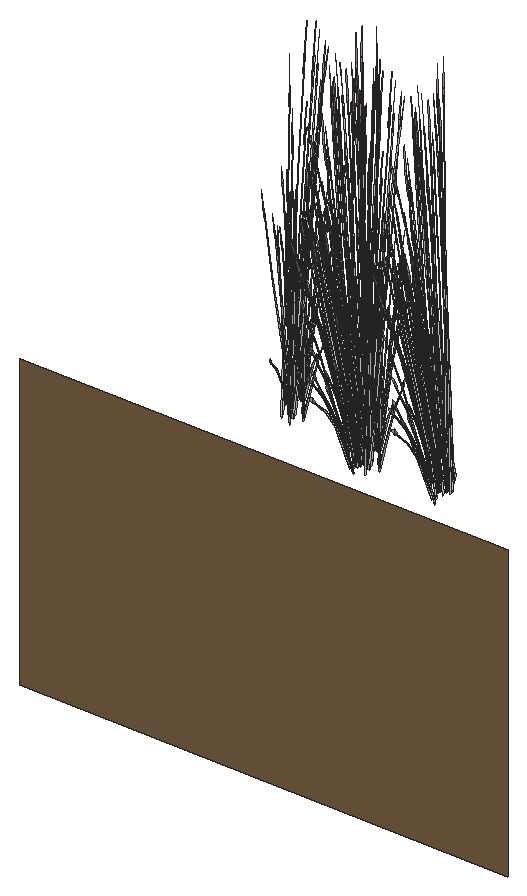
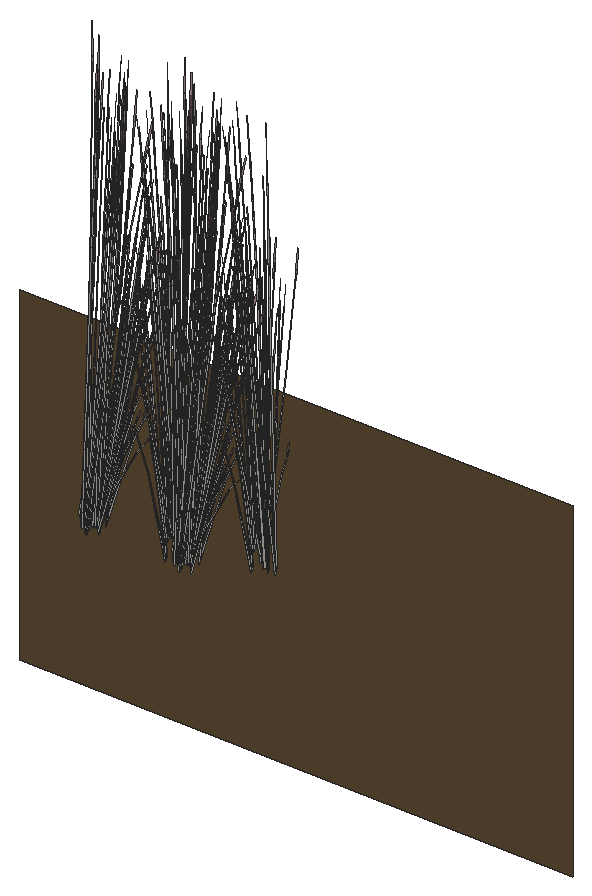
# SketchUp Ruby script. Lengths in inches.
U = 1.inch
M = Sketchup.active_model
def pt(a) = Geom::Point3d.new(a.map { |v| v * U })
def face(e, loops, mat)
  f = e.add_face(loops[0].map { |a| pt(a) })
  loops[1..].each { |l| e.add_face(l.map { |a| pt(a) }).erase! }
  f.material = f.back_material = mat if mat
  f
end
# faces: each face lists its corners as indices into pts; further lists are holes
def faces(e, pts, list, mat = nil) = list.each { |f| face(e, (f[0].is_a?(Array) ? f : [f]).map { |l| l.map { |i| pts[i] } }, mat) }
# xy, xz, yz: faces in a plane at the given z, y or x. An outline is a flat list of corners, or four numbers for a rectangle; further outlines are holes
def ring(l) = l.size == 4 ? [[l[0], l[1]], [l[2], l[1]], [l[2], l[3]], [l[0], l[3]]] : l.each_slice(2).to_a
def flat(e, list, mat, &to3) = list.each { |f| face(e, (f[0].is_a?(Array) ? f : [f]).map { |l| ring(l).map { |u, v| to3.(u, v) } }, mat) }
def xy(e, z, list, mat = nil) = flat(e, list, mat) { |x, y| [x, y, z] }
def xz(e, y, list, mat = nil) = flat(e, list, mat) { |x, z| [x, y, z] }
def yz(e, x, list, mat = nil) = flat(e, list, mat) { |y, z| [x, y, z] }
def lines(e, pts, list) = list.each { |a, b| e.add_line(pt(pts[a]), pt(pts[b])) }
# prism: a flat outline (further loops are holes) pulled along v
def prism(e, loops, v, mat = nil)
  f = face(e, loops, mat); d = Geom::Vector3d.new(v.map { |x| x * U })
  f.pushpull(f.normal.samedirection?(d) ? d.length : -d.length)
end
def box(e, o, s, mat = nil) = prism(e, [[o, [o[0] + s[0], o[1], o[2]], [o[0] + s[0], o[1] + s[1], o[2]], [o[0], o[1] + s[1], o[2]]]], [0, 0, s[2]], mat)
def at(x, y, z, deg = 0) = Geom::Transformation.translation(pt([x, y, z])) * Geom::Transformation.rotation(ORIGIN, Z_AXIS, deg.degrees)
def axes(o, x, y, z) = Geom::Transformation.new([*x, 0, *y, 0, *z, 0, *pt(o).to_a, 1])
def part(name) = M.definitions.add(name)
# library, detail: a bought-in or finely detailed component or shape, given as its bounding box
def library(name, o, s) = part(name).tap { |d| box(d.entities, o, s) }
def detail(e, o, s) = box(e.add_group.entities, o, s)
def put(e, d, t, mat = nil) = e.add_instance(d, t).tap { |i| i.material = mat if mat }
def group(e, t, mat = nil) = e.add_group.tap { |g| g.transformation = t; g.material = mat if mat }.entities
root = M.entities
M.materials.add("LightPink_Translucent").color = [144, 107, 117]
M.materials["LightPink_Translucent"].alpha = 0.75
M.materials.add("Soil_03_1K").color = [122, 96, 67]
c1 = part("blade")
p = [[2.15,0.21,22],[0,0.17,0],[0.09,0.45,0],[2.18,0.31,22],[2.29,0.31,22],[0.38,0.45,0],
  [2.48,0.24,33],[2.49,0.24,33],[2.48,0.22,33]]
faces(c1.entities,p,[[0,1,2,3],[4,5,2,3],[6,3,4,7],[8,0,3,6]])
c2 = part("seeds")
p = [[0.3,-0.1,1.38],[-0.01,-0.03,1.59],[-0.01,-0.03,0.03],[0.14,-0.07,-0.07],[0.29,-0.03,3],[0.15,0.01,3.11]]
faces(c2.entities,p,[[0,1,2,3],[1,0,4,5]],"LightPink_Translucent")
c3 = part("blade with seeds")
put(c3.entities,c1,at(0,0,0))
put(c3.entities,c2,axes([2.4,0.25,30.99],[1.5799,-0.05474,1.17369],[-0.12525,1.92788,0.29478],[-0.07173,-0.02425,1.56792]))
xz(root,0,[[330.57,-48,410.57,0]],"Soil_03_1K")
put(root,c3,axes([368.82,20.52,-9.47],[0.08068,0.14973,1.71376],[-0.3728,0.12606,0.13857],[-0.08426,-0.23506,0.73262]))
put(root,c3,axes([382.24,20.52,-9.33],[0.08068,0.14973,1.71376],[-0.3728,0.12606,0.13857],[-0.08426,-0.23506,0.73262]))
put(root,c3,axes([369.43,19.52,-8.625],[-0.05398,-0.06539,1.74944],[-0.36026,0.04145,-0.27667],[-0.0575,-0.15639,0.14031]))
put(root,c3,axes([382.86,19.52,-8.5],[-0.05398,-0.06539,1.74944],[-0.36026,0.04145,-0.27667],[-0.0575,-0.15639,0.14031]))
put(root,c3,axes([370.27,20.3,-10.75],[-0.10032,0.0944,1.43002],[-0.30046,-0.16522,-0.30754],[0.05569,-0.20547,0.61141]))
put(root,c3,axes([369.8125,20.63,-8.36],[-0.16845,-0.3792,-0.71045],[0.34676,-0.21133,0.08574],[-0.03939,-0.18322,1.00501]))
put(root,c3,axes([383.24,20.63,-8.23],[-0.16845,-0.3792,-0.71045],[0.34676,-0.21133,0.08574],[-0.03939,-0.18322,1.00501]))
put(root,c3,axes([368.72,20.12,-10.75],[-0.02137,0.15256,1.43002],[-0.31245,0.12771,-0.30754],[-0.07303,-0.19719,0.61141]))
put(root,c3,axes([382.14,20.12,-10.62],[-0.02137,0.15256,1.43002],[-0.31245,0.12771,-0.30754],[-0.07303,-0.19719,0.61141]))
put(root,c3,axes([369.52,19.79,-11.85],[-0.0592,0.0168,1.76342],[-0.32738,-0.18913,-0.26939],[0.00549,-0.15776,0.30037]))
put(root,c3,axes([382.95,19.79,-11.72],[-0.0592,0.0168,1.76342],[-0.32738,-0.18913,-0.26939],[0.00549,-0.15776,0.30037]))
put(root,c3,axes([358.04,21,-5.34],[0.00918,-0.43138,-0.71045],[0.38672,0.02897,0.08574],[0.04081,-0.18275,1.00501]))
put(root,c3,axes([370.51,21,-8.36],[0.00918,-0.43138,-0.71045],[0.38672,0.02897,0.08574],[0.04081,-0.18275,1.00501]))
put(root,c3,axes([358.58,20.33,-5.61],[-0.00341,-0.09282,1.74944],[-0.28775,-0.26825,-0.27667],[0.04449,-0.16261,0.14031]))
put(root,c3,axes([371.05,20.33,-8.625],[-0.00341,-0.09282,1.74944],[-0.28775,-0.26825,-0.27667],[0.04449,-0.16261,0.14031]))
put(root,c3,axes([369.84,20.31,-8.82],[0.1064,-0.35863,-0.35414],[0.31043,0.1046,0.4572],[-0.02846,-0.14439,0.87481]))
put(root,c3,axes([383.27,20.31,-8.68],[0.1064,-0.35863,-0.35414],[0.31043,0.1046,0.4572],[-0.02846,-0.14439,0.87481]))
put(root,c3,axes([357.6,20.78,-6.45],[-0.06572,0.16029,1.71376],[-0.27569,-0.33172,0.13857],[0.12437,-0.20675,0.73262]))
put(root,c3,axes([370.08,20.78,-9.47],[-0.06572,0.16029,1.71376],[-0.27569,-0.33172,0.13857],[0.12437,-0.20675,0.73262]))
put(root,c3,axes([370.98,19.99,-8.63],[-0.03584,0.03562,1.77383],[-0.35118,-0.12018,-0.16761],[-0.01271,-0.15545,0.31391]))
put(root,c3,axes([369.6875,20.55,-8.66],[-0.34695,-0.11691,-0.51099],[0.11892,-0.40083,-0.3958],[-0.03181,-0.16138,0.97773]))
put(root,c3,axes([383.11,20.55,-8.53],[-0.34695,-0.11691,-0.51099],[0.11892,-0.40083,-0.3958],[-0.03181,-0.16138,0.97773]))
put(root,c3,axes([369.9,19.55,-10.58],[0.04528,0.27194,1.1486],[-0.25117,-0.15062,0.84392],[0.02703,-0.13924,0.25299]))
put(root,c3,axes([370.4375,20.86,-8.66],[-0.25266,-0.31335,-0.51099],[0.2669,-0.27442,-0.3958],[0.03844,-0.15921,0.97773]))
put(root,c3,axes([369.07,19.31,-8.63],[-0.00658,0.0559,1.77383],[-0.32474,0.20287,-0.16761],[-0.09556,-0.1037,0.31391]))
put(root,c3,axes([382.49,19.31,-8.5],[-0.00658,0.0559,1.77383],[-0.32474,0.20287,-0.16761],[-0.09556,-0.1037,0.31391]))
put(root,c3,axes([368.99,20.3,-8.25],[0.39316,-0.11987,0.53763],[0.06823,0.47021,0.4433],[-0.09247,-0.13858,1.11249]))
put(root,c3,axes([382.42,20.3,-8.12],[0.39316,-0.11987,0.53763],[0.06823,0.47021,0.4433],[-0.09247,-0.13858,1.11249]))
put(root,c3,axes([369.88,20.39,-8.61],[0.34777,0.12192,0.48003],[-0.11892,0.40083,0.3958],[-0.0209,-0.15763,0.9933]))
put(root,c3,axes([369.98,20.53,-8.31],[-0.34538,0.21713,-0.1216],[-0.16972,-0.38536,-0.67495],[-0.04557,-0.16239,1.02557]))
put(root,c3,axes([383.41,20.53,-8.18],[-0.34538,0.21713,-0.1216],[-0.16972,-0.38536,-0.67495],[-0.04557,-0.16239,1.02557]))
put(root,c3,axes([370.7,21.02,-8.31],[-0.3879,-0.02311,-0.1216],[0.0106,-0.43749,-0.67495],[0.02694,-0.1685,1.02557]))
put(root,c3,axes([358.2,20.74,-5.8],[0.23881,-0.24554,-0.35414],[0.22606,0.28036,0.4572],[0.0344,-0.14245,0.87481]))
put(root,c3,axes([370.67,20.74,-8.82],[0.23881,-0.24554,-0.35414],[0.22606,0.28036,0.4572],[0.0344,-0.14245,0.87481]))
put(root,c3,axes([368.61,19.875,-10.58],[0.18411,0.16231,1.1486],[-0.26813,0.09757,0.84392],[-0.05737,-0.12474,0.25299]))
put(root,c3,axes([382.03,19.875,-10.45],[0.18411,0.16231,1.1486],[-0.26813,0.09757,0.84392],[-0.05737,-0.12474,0.25299]))
put(root,c3,axes([369.98,20.36,-8.61],[0.26007,-0.1585,0.0643],[0.12729,0.28902,0.50621],[-0.02512,-0.1274,0.77189]))
put(root,c3,axes([383.4,20.36,-8.48],[0.26007,-0.1585,0.0643],[0.12729,0.28902,0.50621],[-0.02512,-0.1274,0.77189]))
put(root,c3,axes([369.05,20.74,-8.36],[-0.30095,-0.22541,-0.71045],[0.21388,-0.395,0.08574],[-0.10904,-0.13459,1.00501]))
put(root,c3,axes([382.48,20.74,-8.23],[-0.30095,-0.22541,-0.71045],[0.21388,-0.395,0.08574],[-0.10904,-0.13459,1.00501]))
put(root,c3,axes([368.95,20.4375,-8.82],[-0.05451,-0.37564,-0.35414],[0.31161,-0.09919,0.4572],[-0.0837,-0.10765,0.87481]))
put(root,c3,axes([382.375,20.4375,-8.68],[-0.05451,-0.37564,-0.35414],[0.31161,-0.09919,0.4572],[-0.0837,-0.10765,0.87481]))
put(root,c3,axes([369.08,20.4,-8.61],[0.16041,-0.29625,0.0643],[0.22843,0.17248,0.50621],[-0.07385,-0.09498,0.77189]))
put(root,c3,axes([382.51,20.4,-8.48],[0.16041,-0.29625,0.0643],[0.22843,0.17248,0.50621],[-0.07385,-0.09498,0.77189]))
put(root,c3,axes([368.46,20.37,-11.85],[-0.03419,0.06144,1.76342],[-0.3455,0.13246,-0.26939],[-0.08346,-0.12049,0.30037]))
put(root,c3,axes([381.89,20.37,-11.72],[-0.03419,0.06144,1.76342],[-0.3455,0.13246,-0.26939],[-0.08346,-0.12049,0.30037]))
put(root,c3,axes([369.03,22.05,-11.24],[-0.14494,-0.47823,-0.69835],[0.41752,-0.17223,-0.18329],[-0.01602,-0.16194,1.54149]))
put(root,c3,axes([382.46,22.05,-11.11],[-0.14494,-0.47823,-0.69835],[0.41752,-0.17223,-0.18329],[-0.01602,-0.16194,1.54149]))
put(root,c3,axes([368.28,20.98,-9.47],[0.1311,0.08035,1.71376],[-0.27131,0.33708,0.13857],[-0.16909,-0.15206,0.73262]))
put(root,c3,axes([381.7,20.98,-9.33],[0.1311,0.08035,1.71376],[-0.27131,0.33708,0.13857],[-0.16909,-0.15206,0.73262]))
put(root,c3,axes([358.5,20.59,-8.83],[-0.05283,-0.03674,1.76342],[-0.13569,-0.41045,-0.26939],[0.09154,-0.11138,0.30037]))
put(root,c3,axes([370.97,20.59,-11.85],[-0.05283,-0.03674,1.76342],[-0.13569,-0.41045,-0.26939],[0.09154,-0.11138,0.30037]))
put(root,c3,axes([369.88,20.68,-8.29],[-0.1064,0.35863,0.35414],[-0.31043,-0.1046,-0.4572],[-0.02846,-0.14439,0.87481]))
put(root,c3,axes([383.3,20.68,-8.16],[-0.1064,0.35863,0.35414],[-0.31043,-0.1046,-0.4572],[-0.02846,-0.14439,0.87481]))
put(root,c3,axes([368.91,20.75,-8.66],[-0.34827,0.11086,-0.51099],[-0.06092,-0.41983,-0.3958],[-0.09354,-0.12031,0.97773]))
put(root,c3,axes([382.34,20.75,-8.53],[-0.34827,0.11086,-0.51099],[-0.06092,-0.41983,-0.3958],[-0.09354,-0.12031,0.97773]))
put(root,c3,axes([358.2,20.84,-5.59],[0.25132,0.3182,0.48003],[-0.2669,0.27442,0.3958],[0.04636,-0.14929,0.9933]))
put(root,c3,axes([370.67,20.84,-8.61],[0.25132,0.3182,0.48003],[-0.2669,0.27442,0.3958],[0.04636,-0.14929,0.9933]))
put(root,c3,axes([369.16,20.375,-7.91],[-0.23555,0.44708,-0.13619],[-0.34112,-0.25757,-0.75594],[-0.11858,-0.12631,1.14864]))
put(root,c3,axes([382.58,20.375,-7.78],[-0.23555,0.44708,-0.13619],[-0.34112,-0.25757,-0.75594],[-0.11858,-0.12631,1.14864]))
put(root,c3,axes([358.29,20.87,-5.59],[0.29004,0.02173,0.0643],[-0.00795,0.32812,0.50621],[0.03035,-0.12569,0.77189]))
put(root,c3,axes([370.77,20.87,-8.61],[0.29004,0.02173,0.0643],[-0.00795,0.32812,0.50621],[0.03035,-0.12569,0.77189]))
put(root,c3,axes([370.55,21.09,-8.29],[-0.23881,0.24554,0.35414],[-0.22606,-0.28036,-0.4572],[0.0344,-0.14245,0.87481]))
put(root,c3,axes([358.49,21.75,-5.34],[0.18436,-0.36797,-0.71045],[0.32306,0.26151,0.08574],[0.11008,-0.13332,1.00501]))
put(root,c3,axes([370.97,21.75,-8.36],[0.18436,-0.36797,-0.71045],[0.32306,0.26151,0.08574],[0.11008,-0.13332,1.00501]))
put(root,c3,axes([368.98,20.68,-10.97],[-0.22066,-0.46731,0],[0.36918,-0.26061,-0.51607],[0.08408,-0.05936,1.63711]))
put(root,c3,axes([358.49,21.58,-5.64],[-0.09067,-0.42583,-0.51099],[0.34336,-0.07449,-0.3958],[0.0984,-0.11438,0.97773]))
put(root,c3,axes([370.96,21.58,-8.66],[-0.09067,-0.42583,-0.51099],[0.34336,-0.07449,-0.3958],[0.0984,-0.11438,0.97773]))
put(root,c3,axes([369.46,20.12,-11.21],[-0.2439,0.26754,-0.03893],[-0.22348,-0.29302,-0.17649],[-0.01573,-0.08303,0.58215]))
put(root,c3,axes([382.89,20.12,-11.08],[-0.2439,0.26754,-0.03893],[-0.22348,-0.29302,-0.17649],[-0.01573,-0.08303,0.58215]))
put(root,c3,axes([368.25,20.24,-8.625],[-0.07594,-0.00329,1.74944],[-0.24177,0.32918,-0.27667],[-0.129,-0.06726,0.14031]))
put(root,c3,axes([381.68,20.24,-8.5],[-0.07594,-0.00329,1.74944],[-0.24177,0.32918,-0.27667],[-0.129,-0.06726,0.14031]))
put(root,c3,axes([358.65,21.88,-5.29],[-0.32648,-0.25715,-0.1216],[0.18809,-0.3724,-0.67495],[0.09224,-0.12945,1.02557]))
put(root,c3,axes([371.12,21.88,-8.31],[-0.32648,-0.25715,-0.1216],[0.18809,-0.3724,-0.67495],[0.09224,-0.12945,1.02557]))
put(root,c3,axes([369.77,23.29,-10.02],[0.305,0.18805,1.51261],[-0.29879,0.40513,0.59816],[-0.13384,-0.24012,1.26806]))
put(root,c3,axes([383.2,23.29,-9.89],[0.305,0.18805,1.51261],[-0.29879,0.40513,0.59816],[-0.13384,-0.24012,1.26806]))
put(root,c3,axes([369.13,20.74,-8.29],[0.05451,0.37564,0.35414],[-0.31161,0.09919,-0.4572],[-0.0837,-0.10765,0.87481]))
put(root,c3,axes([382.56,20.74,-8.16],[0.05451,0.37564,0.35414],[-0.31161,0.09919,-0.4572],[-0.0837,-0.10765,0.87481]))
put(root,c3,axes([368.18,21.99,-11.32],[0,-0.46636,-0.49651],[0.39487,0,0],[0,-0.10622,1.57504]))
put(root,c3,axes([381.6,21.99,-11.19],[0,-0.46636,-0.49651],[0.39487,0,0],[0,-0.10622,1.57504]))
put(root,c3,axes([356.8,20.61,-8.3],[0.33032,-0.23318,-0.49651],[0.19744,0.41812,0],[0.07523,-0.05311,1.57504]))
put(root,c3,axes([369.28,20.61,-11.32],[0.33032,-0.23318,-0.49651],[0.19744,0.41812,0],[0.07523,-0.05311,1.57504]))
put(root,c3,axes([358.76,21.41,-7.73],[-0.12609,-0.01381,1.43002],[-0.12917,-0.37055,-0.30754],[0.1549,-0.10482,0.61141]))
put(root,c3,axes([371.24,21.41,-10.75],[-0.12609,-0.01381,1.43002],[-0.12917,-0.37055,-0.30754],[0.1549,-0.10482,0.61141]))
put(root,c3,axes([368.2,20.99,-8.25],[0.29147,-0.34417,0.53763],[0.25138,0.3655,0.4433],[-0.13675,-0.06349,1.11249]))
put(root,c3,axes([381.625,20.99,-8.12],[0.29147,-0.34417,0.53763],[0.25138,0.3655,0.4433],[-0.13675,-0.06349,1.11249]))
put(root,c3,axes([359.45,21.77,-5.61],[-0.0461,-0.00354,1.77383],[-0.19143,-0.37951,-0.16761],[0.07688,-0.12478,0.31391]))
put(root,c3,axes([371.93,21.77,-8.63],[-0.0461,-0.00354,1.77383],[-0.19143,-0.37951,-0.16761],[0.07688,-0.12478,0.31391]))
put(root,c3,axes([357.19,21.5625,-8.26],[0.23773,-0.35053,-0.62353],[0.29532,0.31785,-0.16365],[0.09526,-0.08744,1.37633]))
put(root,c3,axes([369.67,21.5625,-11.28],[0.23773,-0.35053,-0.62353],[0.29532,0.31785,-0.16365],[0.09526,-0.08744,1.37633]))
put(root,c3,axes([358.91,20.73,-7.56],[-0.11756,0.2374,1.1486],[-0.10105,-0.31895,0.84392],[0.09709,-0.07992,0.25299]))
put(root,c3,axes([371.38,20.73,-10.58],[-0.11756,0.2374,1.1486],[-0.10105,-0.31895,0.84392],[0.09709,-0.07992,0.25299]))
put(root,c3,axes([358.74,21.62,-5.8],[0.30722,-0.06665,-0.35414],[0.08112,0.381,0.4572],[0.08804,-0.10234,0.87481]))
put(root,c3,axes([371.21,21.62,-8.82],[0.30722,-0.06665,-0.35414],[0.08112,0.381,0.4572],[0.08804,-0.10234,0.87481]))
put(root,c3,axes([368.33,20.99,-8.61],[0.01777,-0.35463,0.0643],[0.26836,0.00972,0.50621],[-0.1028,-0.03711,0.77189]))
put(root,c3,axes([381.76,20.99,-8.48],[0.01777,-0.35463,0.0643],[0.26836,0.00972,0.50621],[-0.1028,-0.03711,0.77189]))
put(root,c3,axes([369.25,22.18,-11.13],[0.17124,-0.42022,-0.44739],[0.35581,0.20224,0.21531],[0,-0.09687,1.43643]))
put(root,c3,axes([382.68,22.18,-11],[0.17124,-0.42022,-0.44739],[0.35581,0.20224,0.21531],[0,-0.09687,1.43643]))
put(root,c3,axes([368.23,21.1,-8.82],[-0.20082,-0.29199,-0.35414],[0.2293,-0.2764,0.4572],[-0.1165,-0.04206,0.87481]))
put(root,c3,axes([381.65,21.1,-8.68],[-0.20082,-0.29199,-0.35414],[0.2293,-0.2764,0.4572],[-0.1165,-0.04206,0.87481]))
put(root,c3,axes([369.41,21.97,-10.68],[-0.04113,-0.53214,-0.29095],[0.42835,-0.03218,-0.50002],[0.07543,-0.07088,1.59708]))
put(root,c3,axes([368.35,22,-11.3125],[0.24637,-0.29097,-0.30978],[0.24637,0.29097,0.30978],[0,-0.09372,1.38974]))
put(root,c3,axes([381.77,22,-11.18],[0.24637,-0.29097,-0.30978],[0.24637,0.29097,0.30978],[0,-0.09372,1.38974]))
put(root,c3,axes([368.25,20.6,-11.21],[-0.10181,0.3808,-0.03893],[-0.31336,-0.11714,-0.17649],[-0.04758,-0.06228,0.58215]))
put(root,c3,axes([381.67,20.6,-11.08],[-0.10181,0.3808,-0.03893],[-0.31336,-0.11714,-0.17649],[-0.04758,-0.06228,0.58215]))
put(root,c3,axes([358.49,21.85,-5.27],[-0.30722,0.06665,0.35414],[-0.08112,-0.381,-0.4572],[0.08804,-0.10234,0.87481]))
put(root,c3,axes([370.96,21.85,-8.29],[-0.30722,0.06665,0.35414],[-0.08112,-0.381,-0.4572],[0.08804,-0.10234,0.87481]))
put(root,c3,axes([369.21,22.53,-10.68],[-0.39748,-0.22252,-0.29095],[0.19139,-0.46966,-0.50002],[-0.01249,-0.11531,1.59708]))
put(root,c3,axes([382.64,22.53,-10.55],[-0.39748,-0.22252,-0.29095],[0.19139,-0.46966,-0.50002],[-0.01249,-0.11531,1.59708]))
put(root,c3,axes([368.08,22.34,-10.97],[-0.44133,0,0],[0,-0.52122,-0.51607],[0,-0.11871,1.63711]))
put(root,c3,axes([381.51,22.34,-10.84],[-0.44133,0,0],[0,-0.52122,-0.51607],[0,-0.11871,1.63711]))
put(root,c3,axes([368.16,21.41,-10.75],[0.06891,0.12984,1.43002],[-0.15879,0.35293,-0.30754],[-0.16304,-0.08436,0.61141]))
put(root,c3,axes([381.58,21.41,-10.62],[0.06891,0.12984,1.43002],[-0.15879,0.35293,-0.30754],[-0.16304,-0.08436,0.61141]))
put(root,c3,axes([369.35,20.79,-11.3125],[0.32928,0.11539,-0.30978],[-0.08291,0.40636,0.30978],[0.06638,-0.04686,1.38974]))
put(root,c3,axes([368.44,21.29,-8.36],[-0.35281,-0.01123,-0.71045],[0.0237,-0.47284,0.08574],[-0.14947,-0.0499,1.00501]))
put(root,c3,axes([381.87,21.29,-8.23],[-0.35281,-0.01123,-0.71045],[0.0237,-0.47284,0.08574],[-0.14947,-0.0499,1.00501]))
put(root,c3,axes([358.77,21.79,-5.59],[0.2423,0.19613,0.0643],[-0.14107,0.2793,0.50621],[0.07768,-0.0903,0.77189]))
put(root,c3,axes([371.24,21.79,-8.61],[0.2423,0.19613,0.0643],[-0.14107,0.2793,0.50621],[0.07768,-0.0903,0.77189]))
put(root,c3,axes([358.7,21.71,-5.59],[0.08753,0.42921,0.48003],[-0.34336,0.07449,0.3958],[0.1012,-0.10094,0.9933]))
put(root,c3,axes([371.17,21.71,-8.61],[0.08753,0.42921,0.48003],[-0.34336,0.07449,0.3958],[0.1012,-0.10094,0.9933]))
put(root,c3,axes([359.625,22.22,-5.61],[0.04898,-0.07104,1.74944],[-0.06269,-0.43574,-0.27667],[0.12289,-0.08262,0.14031]))
put(root,c3,axes([372.1,22.22,-8.625],[0.04898,-0.07104,1.74944],[-0.06269,-0.43574,-0.27667],[0.12289,-0.08262,0.14031]))
put(root,c3,axes([368.42,22.2,-11.01],[-0.32829,0.39208,0.30756],[-0.32849,-0.38796,-0.36492],[-0.01146,-0.11134,1.64885]))
put(root,c3,axes([381.85,22.2,-10.88],[-0.32829,0.39208,0.30756],[-0.32849,-0.38796,-0.36492],[-0.01146,-0.11134,1.64885]))
put(root,c3,axes([367.96,20.52,-8.63],[0.02617,0.04654,1.77383],[-0.12614,0.41836,-0.16761],[-0.12775,0.00303,0.31391]))
put(root,c3,axes([381.39,20.52,-8.5],[0.02617,0.04654,1.77383],[-0.12614,0.41836,-0.16761],[-0.12775,0.00303,0.31391]))
put(root,c3,axes([369.47,22.39,-10.91],[0.39767,0.22603,0.24065],[-0.19139,0.46966,0.50002],[0,-0.10827,1.60543]))
put(root,c3,axes([369.3125,23.02,-10.9],[0.09355,-0.55261,-0.23429],[0.44354,0.09633,0.51271],[-0.0775,-0.07631,1.5644]))
put(root,c3,axes([382.74,23.02,-10.77],[0.09355,-0.55261,-0.23429],[0.44354,0.09633,0.51271],[-0.0775,-0.07631,1.5644]))
put(root,c3,axes([368.32,21.39,-8.66],[-0.25628,0.30892,-0.51099],[-0.22444,-0.32634,-0.3958],[-0.13021,-0.047,0.97773]))
put(root,c3,axes([381.75,21.39,-8.53],[-0.25628,0.30892,-0.51099],[-0.22444,-0.32634,-0.3958],[-0.13021,-0.047,0.97773]))
put(root,c3,axes([368.51,21.25,-8.29],[0.20082,0.29199,0.35414],[-0.2293,0.2764,-0.4572],[-0.1165,-0.04206,0.87481]))
put(root,c3,axes([381.9375,21.25,-8.16],[0.20082,0.29199,0.35414],[-0.2293,0.2764,-0.4572],[-0.1165,-0.04206,0.87481]))
put(root,c3,axes([367.75,21.8,-10.58],[0.22533,-0.03337,1.1486],[-0.14293,0.29403,0.84392],[-0.11135,-0.04411,0.25299]))
put(root,c3,axes([381.17,21.8,-10.45],[0.22533,-0.03337,1.1486],[-0.14293,0.29403,0.84392],[-0.11135,-0.04411,0.25299]))
put(root,c3,axes([369.34,22.07,-10.625],[-0.38326,0.02879,0.44739],[-0.03466,-0.47788,-0.21531],[0.06861,-0.04843,1.43643]))
put(root,c3,axes([368.46,21.07,-8.31],[-0.0189,0.47427,-0.1216],[-0.35781,-0.01296,-0.67495],[-0.13781,-0.03295,1.02557]))
put(root,c3,axes([381.88,21.07,-8.18],[-0.0189,0.47427,-0.1216],[-0.35781,-0.01296,-0.67495],[-0.13781,-0.03295,1.02557]))
put(root,c3,axes([368.35,22.42,-10.86],[0,0.46636,0.49651],[-0.39487,0,0],[0,-0.10622,1.57504]))
put(root,c3,axes([381.77,22.42,-10.73],[0,0.46636,0.49651],[-0.39487,0,0],[0,-0.10622,1.57504]))
put(root,c3,axes([358.66,22.89,-5.29],[-0.17758,-0.42229,-0.1216],[0.31518,-0.20752,-0.67495],[0.13282,-0.05572,1.02557]))
put(root,c3,axes([371.14,22.89,-8.31],[-0.17758,-0.42229,-0.1216],[0.31518,-0.20752,-0.67495],[0.13282,-0.05572,1.02557]))
put(root,c3,axes([358.64,22.52,-5.64],[0.09562,-0.42421,-0.51099],[0.32782,0.1454,-0.3958],[0.13199,-0.0389,0.97773]))
put(root,c3,axes([371.12,22.52,-8.66],[0.09562,-0.42421,-0.51099],[0.32782,0.1454,-0.3958],[0.13199,-0.0389,0.97773]))
put(root,c3,axes([358.125,20.8,-7.95],[0.22066,-0.46731,0],[0.36918,0.26061,-0.51607],[0.08408,0.05936,1.63711]))
put(root,c3,axes([370.6,20.8,-10.97],[0.22066,-0.46731,0],[0.36918,0.26061,-0.51607],[0.08408,0.05936,1.63711]))
put(root,c3,axes([368,21.72,-9.47],[0.14639,-0.01056,1.71376],[-0.09712,0.45778,0.13857],[-0.20862,-0.02831,0.73262]))
put(root,c3,axes([381.43,21.72,-9.33],[0.14639,-0.01056,1.71376],[-0.09712,0.45778,0.13857],[-0.20862,-0.02831,0.73262]))
put(root,c3,axes([369.28,22.8,-11.13],[-0.21202,-0.39143,-0.44739],[0.32115,-0.27564,0.21531],[-0.06861,-0.04843,1.43643]))
put(root,c3,axes([382.71,22.8,-11],[-0.21202,-0.39143,-0.44739],[0.32115,-0.27564,0.21531],[-0.06861,-0.04843,1.43643]))
put(root,c3,axes([369.32,22.24,-10.98],[0.15345,0.52148,0.45755],[-0.43845,0.18134,0.17955],[0.00536,-0.09582,1.58856]))
put(root,c3,axes([382.75,22.24,-10.85],[0.15345,0.52148,0.45755],[-0.43845,0.18134,0.17955],[0.00536,-0.09582,1.58856]))
put(root,c3,axes([359,22.64,-8.34],[-0.22732,0.05597,1.41583],[-0.03618,-0.44548,0.08104],[0.15921,-0.06743,0.80566]))
put(root,c3,axes([371.47,22.64,-11.36],[-0.22732,0.05597,1.41583],[-0.03618,-0.44548,0.08104],[0.15921,-0.06743,0.80566]))
put(root,c3,axes([359.41,22.25,-8.0625],[-0.21881,-0.29821,-0.06488],[0.23965,-0.27324,-0.29416],[0.0679,-0.01924,0.97024]))
put(root,c3,axes([371.88,22.25,-11.08],[-0.21881,-0.29821,-0.06488],[0.23965,-0.27324,-0.29416],[0.0679,-0.01924,0.97024]))
put(root,c3,axes([369.25,22.65,-10.625],[-0.17124,0.42022,0.44739],[-0.35581,-0.20224,-0.21531],[0,-0.09687,1.43643]))
put(root,c3,axes([382.67,22.65,-10.49],[-0.17124,0.42022,0.44739],[-0.35581,-0.20224,-0.21531],[0,-0.09687,1.43643]))
put(root,c3,axes([369.875,22.29,-11.14],[0,-0.53961,0],[0.44133,0,0],[0,0,1.79456]))
put(root,c3,axes([383.3,22.29,-11.01],[0,-0.53961,0],[0.44133,0,0],[0,0,1.79456]))
put(root,c3,axes([357.9375,21.04,-7.84],[-0.33032,-0.23318,0.49651],[0.19744,-0.41812,0],[0.07523,0.05311,1.57504]))
put(root,c3,axes([370.41,21.04,-10.86],[-0.33032,-0.23318,0.49651],[0.19744,-0.41812,0],[0.07523,0.05311,1.57504]))
put(root,c3,axes([358.58,22.68,-5.34],[0.31014,-0.20596,-0.71045],[0.17284,0.42397,0.08574],[0.14985,-0.04816,1.00501]))
put(root,c3,axes([371.06,22.68,-8.36],[0.31014,-0.20596,-0.71045],[0.17284,0.42397,0.08574],[0.14985,-0.04816,1.00501]))
put(root,c3,axes([369.09,22.95,-11.28],[-0.36714,-0.07646,-0.62353],[0.07747,-0.47163,-0.16365],[-0.10956,-0.05715,1.37633]))
put(root,c3,axes([382.52,22.95,-11.15],[-0.36714,-0.07646,-0.62353],[0.07747,-0.47163,-0.16365],[-0.10956,-0.05715,1.37633]))
put(root,c3,axes([369.67,21.95,-10.98],[-0.29264,0.42323,0.45755],[-0.34767,-0.3736,0.17955],[0.07055,-0.04224,1.58856]))
put(root,c3,axes([369.99,22.71,-11.04],[-0.32829,-0.4014,-0.06131],[0.32849,-0.40164,0],[-0.01146,-0.01402,1.75571]))
put(root,c3,axes([383.41,22.71,-10.91],[-0.32829,-0.4014,-0.06131],[0.32849,-0.40164,0],[-0.01146,-0.01402,1.75571]))
put(root,c3,axes([369.16,21.25,-10.87],[-0.10196,0.46348,0.17642],[-0.3731,-0.13116,0.35086],[0.06445,-0.00226,1.60407]))
put(root,c3,axes([358.54,22.76,-5.27],[-0.29332,-0.1301,0.35414],[0.08555,-0.37955,-0.4572],[0.11809,-0.0348,0.87481]))
put(root,c3,axes([371.01,22.76,-8.29],[-0.29332,-0.1301,0.35414],[0.08555,-0.37955,-0.4572],[0.11809,-0.0348,0.87481]))
put(root,c3,axes([367.94,22.07,-8.61],[0.09971,-0.42522,0.48003],[0.32782,0.1454,0.3958],[-0.12892,0.02555,0.9933]))
put(root,c3,axes([381.37,22.07,-8.48],[0.09971,-0.42522,0.48003],[0.32782,0.1454,0.3958],[-0.12892,0.02555,0.9933]))
put(root,c3,axes([356.53,21.625,-8.73],[-0.3474,0.18671,1.28929],[-0.11057,-0.53572,0.50096],[0.21332,0.00891,1.46642]))
put(root,c3,axes([369.01,21.625,-11.75],[-0.3474,0.18671,1.28929],[-0.11057,-0.53572,0.50096],[0.21332,0.00891,1.46642]))
put(root,c3,axes([357.46,21.77,-7.71],[0.06809,-0.4162,0.1448],[0.33266,0.07225,-0.41347],[0.06054,0.04274,1.26744]))
put(root,c3,axes([369.9375,21.77,-10.73],[0.06809,-0.4162,0.1448],[0.33266,0.07225,-0.41347],[0.06054,0.04274,1.26744]))
put(root,c3,axes([367.92,21.95,-8.61],[-0.12963,-0.31798,0.0643],[0.23638,-0.15564,0.50621],[-0.1042,0.03071,0.77189]))
put(root,c3,axes([381.34,21.95,-8.48],[-0.12963,-0.31798,0.0643],[0.23638,-0.15564,0.50621],[-0.1042,0.03071,0.77189]))
put(root,c3,axes([369.36,22.75,-10.98],[0.44609,0.09826,0.45755],[-0.09078,0.55493,0.17955],[-0.06519,-0.05359,1.58856]))
put(root,c3,axes([382.79,22.75,-10.85],[0.44609,0.09826,0.45755],[-0.09078,0.55493,0.17955],[-0.06519,-0.05359,1.58856]))
put(root,c3,axes([359.24,22.35,-8.83],[-0.01845,-0.0708,1.76342],[0.12793,-0.41416,-0.26939],[0.12905,-0.00596,0.30037]))
put(root,c3,axes([371.72,22.35,-11.85],[-0.01845,-0.0708,1.76342],[0.12793,-0.41416,-0.26939],[0.12905,-0.00596,0.30037]))
put(root,c3,axes([367.91,22.28,-11.85],[0.00895,0.0735,1.76342],[-0.18044,0.38382,-0.26939],[-0.12817,-0.01935,0.30037]))
put(root,c3,axes([381.34,22.28,-11.72],[0.00895,0.0735,1.76342],[-0.18044,0.38382,-0.26939],[-0.12817,-0.01935,0.30037]))
put(root,c3,axes([369.8,21.875,-10.625],[-0.21202,-0.39143,0.44739],[0.32115,-0.27564,-0.21531],[0.06861,0.04843,1.43643]))
put(root,c3,axes([368.7,23.66,-11.3125],[-0.08291,-0.40636,-0.30978],[0.32928,-0.11539,0.30978],[-0.06638,-0.04686,1.38974]))
put(root,c3,axes([382.125,23.66,-11.18],[-0.08291,-0.40636,-0.30978],[0.32928,-0.11539,0.30978],[-0.06638,-0.04686,1.38974]))
put(root,c3,axes([369.125,23.64,-10.87],[0.37926,-0.12378,0.17642],[0.09365,0.46065,0.35086],[-0.03382,-0.06712,1.60407]))
put(root,c3,axes([382.55,23.64,-10.74],[0.37926,-0.12378,0.17642],[0.09365,0.46065,0.35086],[-0.03382,-0.06712,1.60407]))
put(root,c3,axes([357.43,21.9,-7.66],[0.35635,-0.30962,-0.29095],[0.23697,0.43749,-0.50002],[0.08792,0.04443,1.59708]))
put(root,c3,axes([369.9,21.9,-10.68],[0.35635,-0.30962,-0.29095],[0.23697,0.43749,-0.50002],[0.08792,0.04443,1.59708]))
put(root,c3,axes([358.85,22.72,-5.8],[0.29332,0.1301,-0.35414],[-0.08555,0.37955,0.4572],[0.11809,-0.0348,0.87481]))
put(root,c3,axes([371.32,22.72,-8.82],[0.29332,0.1301,-0.35414],[-0.08555,0.37955,0.4572],[0.11809,-0.0348,0.87481]))
put(root,c3,axes([368.61,23.84,-11.32],[-0.33032,-0.23318,-0.49651],[0.19744,-0.41812,0],[-0.07523,-0.05311,1.57504]))
put(root,c3,axes([382.03,23.84,-11.19],[-0.33032,-0.23318,-0.49651],[0.19744,-0.41812,0],[-0.07523,-0.05311,1.57504]))
put(root,c3,axes([358.33,21.08,-8.3],[0.33032,0.23318,-0.49651],[-0.19744,0.41812,0],[0.07523,0.05311,1.57504]))
put(root,c3,axes([370.8,21.08,-11.32],[0.33032,0.23318,-0.49651],[-0.19744,0.41812,0],[0.07523,0.05311,1.57504]))
put(root,c3,axes([367.875,22.11,-8.82],[-0.29332,-0.1301,-0.35414],[0.08555,-0.37955,0.4572],[-0.11809,0.0348,0.87481]))
put(root,c3,axes([381.3,22.11,-8.68],[-0.29332,-0.1301,-0.35414],[0.08555,-0.37955,0.4572],[-0.11809,0.0348,0.87481]))
put(root,c3,axes([370.18,22.41,-11.14],[0.39487,0,0],[0,0.48281,0],[0,0,1.78407]))
put(root,c3,axes([369.51,23.02,-10.68],[-0.35635,0.30962,-0.29095],[-0.23697,-0.43749,-0.50002],[-0.08792,-0.04443,1.59708]))
put(root,c3,axes([382.93,23.02,-10.55],[-0.35635,0.30962,-0.29095],[-0.23697,-0.43749,-0.50002],[-0.08792,-0.04443,1.59708]))
put(root,c3,axes([370.29,21.28,-10.87],[-0.37926,0.12378,0.17642],[-0.09365,-0.46065,0.35086],[0.03382,0.06712,1.60407]))
put(root,c3,axes([358.05,22.25,-6.45],[-0.14639,0.01056,1.71376],[0.09712,-0.45778,0.13857],[0.20862,0.02831,0.73262]))
put(root,c3,axes([370.52,22.25,-9.47],[-0.14639,0.01056,1.71376],[0.09712,-0.45778,0.13857],[0.20862,0.02831,0.73262]))
put(root,c3,axes([358.24,21.25,-8.29],[0.08291,0.40636,-0.30978],[-0.32928,0.11539,0.30978],[0.06638,0.04686,1.38974]))
